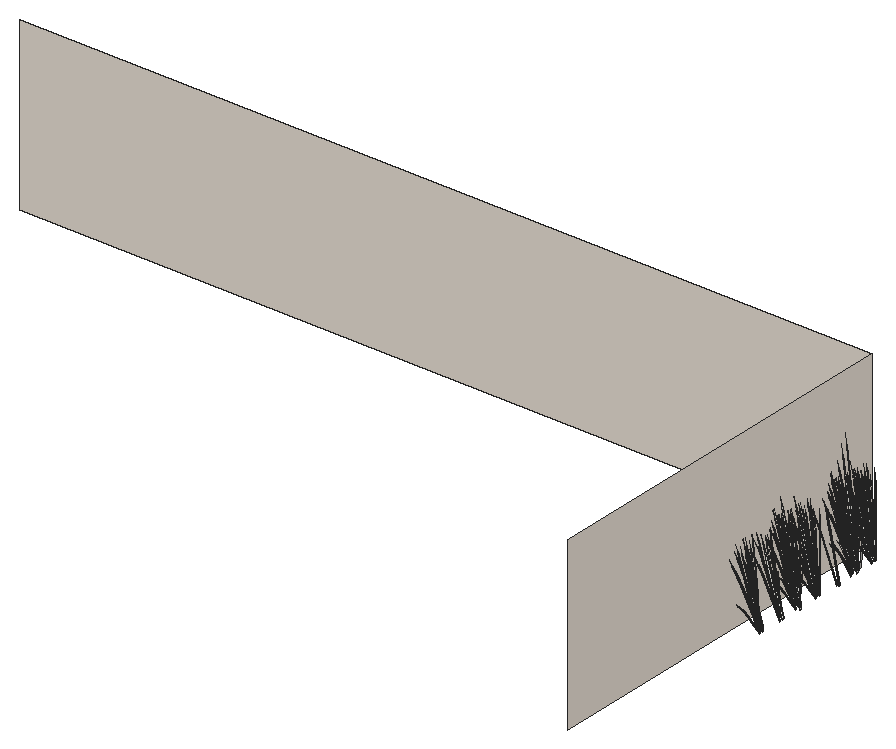
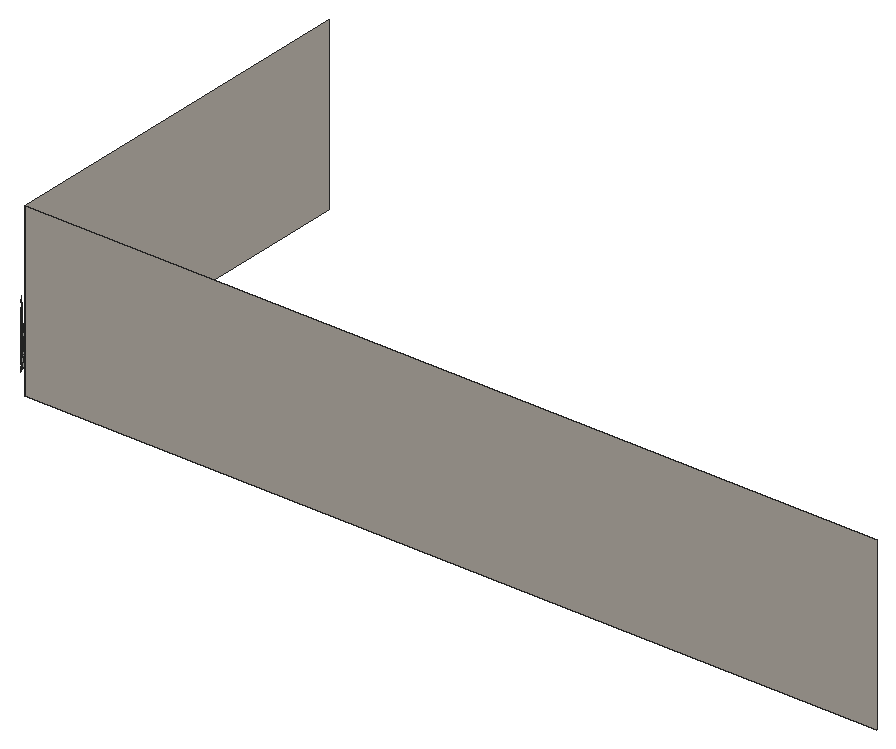
# SketchUp Ruby script. Lengths in inches.
U = 1.inch
M = Sketchup.active_model
def pt(a) = Geom::Point3d.new(a.map { |v| v * U })
def face(e, loops, mat)
  f = e.add_face(loops[0].map { |a| pt(a) })
  loops[1..].each { |l| e.add_face(l.map { |a| pt(a) }).erase! }
  f.material = f.back_material = mat if mat
  f
end
# faces: each face lists its corners as indices into pts; further lists are holes
def faces(e, pts, list, mat = nil) = list.each { |f| face(e, (f[0].is_a?(Array) ? f : [f]).map { |l| l.map { |i| pts[i] } }, mat) }
# xy, xz, yz: faces in a plane at the given z, y or x. An outline is a flat list of corners, or four numbers for a rectangle; further outlines are holes
def ring(l) = l.size == 4 ? [[l[0], l[1]], [l[2], l[1]], [l[2], l[3]], [l[0], l[3]]] : l.each_slice(2).to_a
def flat(e, list, mat, &to3) = list.each { |f| face(e, (f[0].is_a?(Array) ? f : [f]).map { |l| ring(l).map { |u, v| to3.(u, v) } }, mat) }
def xy(e, z, list, mat = nil) = flat(e, list, mat) { |x, y| [x, y, z] }
def xz(e, y, list, mat = nil) = flat(e, list, mat) { |x, z| [x, y, z] }
def yz(e, x, list, mat = nil) = flat(e, list, mat) { |y, z| [x, y, z] }
def lines(e, pts, list) = list.each { |a, b| e.add_line(pt(pts[a]), pt(pts[b])) }
# prism: a flat outline (further loops are holes) pulled along v
def prism(e, loops, v, mat = nil)
  f = face(e, loops, mat); d = Geom::Vector3d.new(v.map { |x| x * U })
  f.pushpull(f.normal.samedirection?(d) ? d.length : -d.length)
end
def box(e, o, s, mat = nil) = prism(e, [[o, [o[0] + s[0], o[1], o[2]], [o[0] + s[0], o[1] + s[1], o[2]], [o[0], o[1] + s[1], o[2]]]], [0, 0, s[2]], mat)
def at(x, y, z, deg = 0) = Geom::Transformation.translation(pt([x, y, z])) * Geom::Transformation.rotation(ORIGIN, Z_AXIS, deg.degrees)
def axes(o, x, y, z) = Geom::Transformation.new([*x, 0, *y, 0, *z, 0, *pt(o).to_a, 1])
def part(name) = M.definitions.add(name)
# library, detail: a bought-in or finely detailed component or shape, given as its bounding box
def library(name, o, s) = part(name).tap { |d| box(d.entities, o, s) }
def detail(e, o, s) = box(e.add_group.entities, o, s)
def put(e, d, t, mat = nil) = e.add_instance(d, t).tap { |i| i.material = mat if mat }
def group(e, t, mat = nil) = e.add_group.tap { |g| g.transformation = t; g.material = mat if mat }.entities
root = M.entities
M.materials.add("LightPink_Translucent").color = [144, 107, 117]
M.materials["LightPink_Translucent"].alpha = 0.75
M.materials.add("Marble_01_1K").color = [230, 221, 211]
c1 = part("blade")
p = [[2.15,0.21,22],[0,0.17,0],[0.09,0.45,0],[2.18,0.31,22],[2.29,0.31,22],[0.38,0.45,0],
  [2.48,0.24,33],[2.49,0.24,33],[2.48,0.22,33]]
faces(c1.entities,p,[[0,1,2,3],[4,5,2,3],[6,3,4,7],[8,0,3,6]])
c2 = part("seeds")
p = [[0.3,-0.1,1.38],[-0.01,-0.03,1.59],[-0.01,-0.03,0.03],[0.14,-0.07,-0.07],[0.29,-0.03,3],[0.15,0.01,3.11]]
faces(c2.entities,p,[[0,1,2,3],[1,0,4,5]],"LightPink_Translucent")
c3 = part("blade with seeds")
put(c3.entities,c1,at(0,0,0))
put(c3.entities,c2,axes([2.4,0.25,30.99],[1.5799,-0.05474,1.17369],[-0.12525,1.92788,0.29478],[-0.07173,-0.02425,1.56792]))
xz(root,432,[[0,-12,390,66]],"Marble_01_1K")
yz(root,390,[[258,-12,432,66]],"Marble_01_1K")
put(root,c3,axes([400.06,408.33,-8.39],[0.21212,-0.01231,1.59586],[-0.14072,0.53355,0.12904],[-0.3023,-0.033,0.68222]))
put(root,c3,axes([400.15,409.27,-8.39],[0.17745,-0.11497,1.59586],[0.14939,0.53127,0.12904],[-0.27857,0.12007,0.68222]))
put(root,c3,axes([399.6,410.18,-9.59],[0.17773,0.04462,1.33163],[0.11455,0.45576,-0.28638],[-0.24142,0.08531,0.56934]))
put(root,c3,axes([400.86,374.66,-8.39],[0.21212,-0.01231,1.59586],[-0.14072,0.53355,0.12904],[-0.3023,-0.033,0.68222]))
put(root,c3,axes([401.17,408.72,-8.89],[0.14537,-0.07863,1.64882],[0.05013,0.549,0.12904],[-0.31487,0.07285,0.5893]))
put(root,c3,axes([401.01,417.9375,-8.39],[0.21212,-0.01231,1.59586],[-0.14072,0.53355,0.12904],[-0.3023,-0.033,0.68222]))
put(root,c3,axes([401.14,385.52,-8.39],[0.21212,-0.01231,1.59586],[-0.14072,0.53355,0.12904],[-0.3023,-0.033,0.68222]))
put(root,c3,axes([399.61,409.09,-7.61],[-0.08351,0.07057,1.62908],[0.0071,0.51561,-0.25764],[-0.19143,0.06705,0.13065]))
put(root,c3,axes([400.69,407.84,-7.36],[-0.51122,-0.01309,-0.66157],[0.03434,-0.5511,0.07984],[-0.21658,-0.05816,0.93586]))
put(root,c3,axes([400.28,407.97,-9.59],[0.09985,0.15133,1.33163],[-0.23008,0.41134,-0.28638],[-0.23625,-0.09832,0.56934]))
put(root,c3,axes([399.875,408.79,-7.78],[-0.42502,-0.15163,-0.32977],[0.12396,-0.44238,0.42575],[-0.17112,0.04056,0.81462]))
put(root,c3,axes([400.95,375.6,-8.39],[0.17745,-0.11497,1.59586],[0.14939,0.53127,0.12904],[-0.27857,0.12007,0.68222]))
put(root,c3,axes([400.46,407.48,-8.39],[0.18996,0.09365,1.59586],[-0.39312,0.39287,0.12904],[-0.24502,-0.17723,0.68222]))
put(root,c3,axes([400.4,376.51,-9.59],[0.17773,0.04462,1.33163],[0.11455,0.45576,-0.28638],[-0.24142,0.08531,0.56934]))
put(root,c3,axes([401.1,418.875,-8.39],[0.17745,-0.11497,1.59586],[0.14939,0.53127,0.12904],[-0.27857,0.12007,0.68222]))
put(root,c3,axes([398.68,409.61,-7.62],[0.06527,0.01458,1.65179],[0.20191,0.48025,-0.15608],[-0.1336,0.12605,0.29231]))
put(root,c3,axes([400.16,409.02,-7.64],[-0.13855,0.49442,-0.47583],[-0.47502,-0.16947,-0.36857],[-0.19125,0.04534,0.91046]))
put(root,c3,axes([400.55,419.78,-9.59],[0.17773,0.04462,1.33163],[0.11455,0.45576,-0.28638],[-0.24142,0.08531,0.56934]))
put(root,c3,axes([401.23,386.46,-8.39],[0.17745,-0.11497,1.59586],[0.14939,0.53127,0.12904],[-0.27857,0.12007,0.68222]))
put(root,c3,axes([401.97,375.05,-8.89],[0.14537,-0.07863,1.64882],[0.05013,0.549,0.12904],[-0.31487,0.07285,0.5893]))
put(root,c3,axes([400.52,407.95,-7.64],[-0.37135,0.36005,-0.47583],[-0.32522,-0.38035,-0.36857],[-0.18868,-0.05478,0.91046]))
put(root,c3,axes([399.93,408.99,-10.61],[0.01297,0.08566,1.6421],[-0.26146,0.44735,-0.25086],[-0.18572,-0.02255,0.2797]))
put(root,c3,axes([400.68,387.37,-9.59],[0.17773,0.04462,1.33163],[0.11455,0.45576,-0.28638],[-0.24142,0.08531,0.56934]))
put(root,c3,axes([402.12,418.32,-8.89],[0.14537,-0.07863,1.64882],[0.05013,0.549,0.12904],[-0.31487,0.07285,0.5893]))
put(root,c3,axes([400,406.94,-7.62],[0.03791,0.05424,1.65179],[-0.18278,0.48761,-0.15608],[-0.18511,0.00353,0.29231]))
put(root,c3,axes([401.91,352.82,-8.39],[0.21212,-0.01231,1.59586],[-0.14072,0.53355,0.12904],[-0.3023,-0.033,0.68222]))
put(root,c3,axes([399.23,411.13,-9.42],[0.21313,-0.24635,1.06958],[0.0841,0.38999,0.78586],[-0.15402,0.06983,0.23558]))
put(root,c3,axes([402.25,385.91,-8.89],[0.14537,-0.07863,1.64882],[0.05013,0.549,0.12904],[-0.31487,0.07285,0.5893]))
put(root,c3,axes([400.42,406.62,-7.61],[-0.11004,-0.00384,1.62908],[-0.35032,0.38367,-0.25764],[-0.18692,-0.07839,0.13065]))
put(root,c3,axes([400.41,375.41,-7.61],[-0.08351,0.07057,1.62908],[0.0071,0.51561,-0.25764],[-0.19143,0.06705,0.13065]))
put(root,c3,axes([401.5,374.17,-7.36],[-0.51122,-0.01309,-0.66157],[0.03434,-0.5511,0.07984],[-0.21658,-0.05816,0.93586]))
put(root,c3,axes([399.97,408.74,-7.59],[0.14449,-0.4956,0.447],[0.47502,0.16947,0.36857],[-0.1868,0.02978,0.92496]))
put(root,c3,axes([401.09,374.3,-9.59],[0.09985,0.15133,1.33163],[-0.23008,0.41134,-0.28638],[-0.23625,-0.09832,0.56934]))
put(root,c3,axes([400.14,408.6,-7.3125],[0.25732,0.49218,-0.11324],[-0.45669,0.24187,-0.62851],[-0.19245,0.06494,0.95501]))
put(root,c3,axes([400.72,407.57,-7.3125],[-0.02738,0.55277,-0.11324],[-0.51847,-0.01511,-0.62851],[-0.19968,-0.0384,0.95501]))
put(root,c3,axes([400.56,418.6875,-7.61],[-0.08351,0.07057,1.62908],[0.0071,0.51561,-0.25764],[-0.19143,0.06705,0.13065]))
put(root,c3,axes([400.39,407.61,-7.78],[-0.29098,-0.34031,-0.32977],[0.33226,-0.32215,0.42575],[-0.16881,-0.04902,0.81462]))
put(root,c3,axes([400.68,375.12,-7.78],[-0.42502,-0.15163,-0.32977],[0.12396,-0.44238,0.42575],[-0.17112,0.04056,0.81462]))
put(root,c3,axes([401.65,417.44,-7.36],[-0.51122,-0.01309,-0.66157],[0.03434,-0.5511,0.07984],[-0.21658,-0.05816,0.93586]))
put(root,c3,axes([399.9375,408.61,-7.6],[-0.18783,-0.37061,0.05988],[0.34252,-0.1814,0.47138],[-0.15099,0.03579,0.71878]))
put(root,c3,axes([401.27,373.81,-8.39],[0.18996,0.09365,1.59586],[-0.39312,0.39287,0.12904],[-0.24502,-0.17723,0.68222]))
put(root,c3,axes([400.8,409.63,-8.39],[0.12773,-0.16701,1.59586],[0.32252,0.4508,0.12904],[-0.22121,0.20529,0.68222]))
put(root,c3,axes([401.23,417.57,-9.59],[0.09985,0.15133,1.33163],[-0.23008,0.41134,-0.28638],[-0.23625,-0.09832,0.56934]))
put(root,c3,axes([400.03,410.07,-7.78],[-0.44516,0.07768,-0.32977],[-0.11755,-0.44407,0.42575],[-0.12757,0.11927,0.81462]))
put(root,c3,axes([400.69,386.27,-7.61],[-0.08351,0.07057,1.62908],[0.0071,0.51561,-0.25764],[-0.19143,0.06705,0.13065]))
put(root,c3,axes([401.78,385.03,-7.36],[-0.51122,-0.01309,-0.66157],[0.03434,-0.5511,0.07984],[-0.21658,-0.05816,0.93586]))
put(root,c3,axes([400.82,418.39,-7.78],[-0.42502,-0.15163,-0.32977],[0.12396,-0.44238,0.42575],[-0.17112,0.04056,0.81462]))
put(root,c3,axes([399.79,411.39,-10.61],[0.0686,0.0543,1.6421],[0.11632,0.50315,-0.25086],[-0.15204,0.10729,0.2797]))
put(root,c3,axes([401.41,417.08,-8.39],[0.18996,0.09365,1.59586],[-0.39312,0.39287,0.12904],[-0.24502,-0.17723,0.68222]))
put(root,c3,axes([401.37,385.16,-9.59],[0.09985,0.15133,1.33163],[-0.23008,0.41134,-0.28638],[-0.23625,-0.09832,0.56934]))
put(root,c3,axes([399.6875,408.43,-9.42],[0.3265,-0.03889,1.06958],[-0.20711,0.3427,0.78586],[-0.16135,-0.05141,0.23558]))
put(root,c3,axes([399.48,375.9375,-7.62],[0.06527,0.01458,1.65179],[0.20191,0.48025,-0.15608],[-0.1336,0.12605,0.29231]))
put(root,c3,axes([400.97,375.35,-7.64],[-0.13855,0.49442,-0.47583],[-0.47502,-0.16947,-0.36857],[-0.19125,0.04534,0.91046]))
put(root,c3,axes([402.43,364.02,-8.39],[0.21212,-0.01231,1.59586],[-0.14072,0.53355,0.12904],[-0.3023,-0.033,0.68222]))
put(root,c3,axes([402,353.75,-8.39],[0.17745,-0.11497,1.59586],[0.14939,0.53127,0.12904],[-0.27857,0.12007,0.68222]))
put(root,c3,axes([400.96,385.98,-7.78],[-0.42502,-0.15163,-0.32977],[0.12396,-0.44238,0.42575],[-0.17112,0.04056,0.81462]))
put(root,c3,axes([401.55,384.66,-8.39],[0.18996,0.09365,1.59586],[-0.39312,0.39287,0.12904],[-0.24502,-0.17723,0.68222]))
put(root,c3,axes([401.33,374.28,-7.64],[-0.37135,0.36005,-0.47583],[-0.32522,-0.38035,-0.36857],[-0.18868,-0.05478,0.91046]))
put(root,c3,axes([400.73,375.32,-10.61],[0.01297,0.08566,1.6421],[-0.26146,0.44735,-0.25086],[-0.18572,-0.02255,0.2797]))
put(root,c3,axes([399.63,419.21,-7.62],[0.06527,0.01458,1.65179],[0.20191,0.48025,-0.15608],[-0.1336,0.12605,0.29231]))
put(root,c3,axes([400.09,409.97,-7.59],[-0.12683,-0.50025,0.447],[0.49754,-0.08682,0.36857],[-0.14663,0.11765,0.92496]))
put(root,c3,axes([401.12,418.62,-7.64],[-0.13855,0.49442,-0.47583],[-0.47502,-0.16947,-0.36857],[-0.19125,0.04534,0.91046]))
put(root,c3,axes([401.45,354.66,-9.59],[0.17773,0.04462,1.33163],[0.11455,0.45576,-0.28638],[-0.24142,0.08531,0.56934]))
put(root,c3,axes([400.34,407.48,-7.26],[0.42234,-0.40113,0.50064],[0.36424,0.42599,0.4128],[-0.19815,-0.07399,1.03595]))
put(root,c3,axes([401.48,417.55,-7.64],[-0.37135,0.36005,-0.47583],[-0.32522,-0.38035,-0.36857],[-0.18868,-0.05478,0.91046]))
put(root,c3,axes([400.81,373.27,-7.62],[0.03791,0.05424,1.65179],[-0.18278,0.48761,-0.15608],[-0.18511,0.00353,0.29231]))
put(root,c3,axes([400.875,418.59,-10.61],[0.01297,0.08566,1.6421],[-0.26146,0.44735,-0.25086],[-0.18572,-0.02255,0.2797]))
put(root,c3,axes([399.76,386.79,-7.62],[0.06527,0.01458,1.65179],[0.20191,0.48025,-0.15608],[-0.1336,0.12605,0.29231]))
put(root,c3,axes([399.99,409.875,-7.6],[-0.35109,-0.22859,0.05988],[0.2044,-0.32553,0.47138],[-0.11256,0.10524,0.71878]))
put(root,c3,axes([401.25,386.2,-7.64],[-0.13855,0.49442,-0.47583],[-0.47502,-0.16947,-0.36857],[-0.19125,0.04534,0.91046]))
put(root,c3,axes([403.02,353.2,-8.89],[0.14537,-0.07863,1.64882],[0.05013,0.549,0.12904],[-0.31487,0.07285,0.5893]))
put(root,c3,axes([400.03,377.46,-9.42],[0.21313,-0.24635,1.06958],[0.0841,0.38999,0.78586],[-0.15402,0.06983,0.23558]))
put(root,c3,axes([401.61,385.14,-7.64],[-0.37135,0.36005,-0.47583],[-0.32522,-0.38035,-0.36857],[-0.18868,-0.05478,0.91046]))
put(root,c3,axes([401.23,372.94,-7.61],[-0.11004,-0.00384,1.62908],[-0.35032,0.38367,-0.25764],[-0.18692,-0.07839,0.13065]))
put(root,c3,axes([401.01,386.17,-10.61],[0.01297,0.08566,1.6421],[-0.26146,0.44735,-0.25086],[-0.18572,-0.02255,0.2797]))
put(root,c3,axes([400.95,416.54,-7.62],[0.03791,0.05424,1.65179],[-0.18278,0.48761,-0.15608],[-0.18511,0.00353,0.29231]))
put(root,c3,axes([400.7,410.04,-8.39],[0.09522,-0.18683,1.59586],[0.39947,0.38663,0.12904],[-0.18021,0.24097,0.68222]))
put(root,c3,axes([400.78,375.07,-7.59],[0.14449,-0.4956,0.447],[0.47502,0.16947,0.36857],[-0.1868,0.02978,0.92496]))
put(root,c3,axes([400.18,420.73,-9.42],[0.21313,-0.24635,1.06958],[0.0841,0.38999,0.78586],[-0.15402,0.06983,0.23558]))
put(root,c3,axes([400.95,374.92,-7.3125],[0.25732,0.49218,-0.11324],[-0.45669,0.24187,-0.62851],[-0.19245,0.06494,0.95501]))
put(root,c3,axes([401.09,384.13,-7.62],[0.03791,0.05424,1.65179],[-0.18278,0.48761,-0.15608],[-0.18511,0.00353,0.29231]))
put(root,c3,axes([401.375,416.22,-7.61],[-0.11004,-0.00384,1.62908],[-0.35032,0.38367,-0.25764],[-0.18692,-0.07839,0.13065]))
put(root,c3,axes([402.52,364.96,-8.39],[0.17745,-0.11497,1.59586],[0.14939,0.53127,0.12904],[-0.27857,0.12007,0.68222]))
put(root,c3,axes([401.52,373.9,-7.3125],[-0.02738,0.55277,-0.11324],[-0.51847,-0.01511,-0.62851],[-0.19968,-0.0384,0.95501]))
put(root,c3,axes([401.19,373.9375,-7.78],[-0.29098,-0.34031,-0.32977],[0.33226,-0.32215,0.42575],[-0.16881,-0.04902,0.81462]))
put(root,c3,axes([400.74,374.93,-7.6],[-0.18783,-0.37061,0.05988],[0.34252,-0.1814,0.47138],[-0.15099,0.03579,0.71878]))
put(root,c3,axes([400.32,408.74,-7.3],[0.42502,0.15163,0.32977],[-0.12396,0.44238,-0.42575],[-0.17112,0.04056,0.81462]))
put(root,c3,axes([400.31,388.32,-9.42],[0.21313,-0.24635,1.06958],[0.0841,0.38999,0.78586],[-0.15402,0.06983,0.23558]))
put(root,c3,axes([400.92,418.34,-7.59],[0.14449,-0.4956,0.447],[0.47502,0.16947,0.36857],[-0.1868,0.02978,0.92496]))
put(root,c3,axes([401.6,375.96,-8.39],[0.12773,-0.16701,1.59586],[0.32252,0.4508,0.12904],[-0.22121,0.20529,0.68222]))
put(root,c3,axes([400.83,376.4,-7.78],[-0.44516,0.07768,-0.32977],[-0.11755,-0.44407,0.42575],[-0.12757,0.11927,0.81462]))
put(root,c3,axes([401.97,365.86,-9.59],[0.17773,0.04462,1.33163],[0.11455,0.45576,-0.28638],[-0.24142,0.08531,0.56934]))
put(root,c3,axes([401.46,353.57,-7.61],[-0.08351,0.07057,1.62908],[0.0071,0.51561,-0.25764],[-0.19143,0.06705,0.13065]))
put(root,c3,axes([401.09,418.2,-7.3125],[0.25732,0.49218,-0.11324],[-0.45669,0.24187,-0.62851],[-0.19245,0.06494,0.95501]))
put(root,c3,axes([401.51,383.8,-7.61],[-0.11004,-0.00384,1.62908],[-0.35032,0.38367,-0.25764],[-0.18692,-0.07839,0.13065]))
put(root,c3,axes([402.55,352.32,-7.36],[-0.51122,-0.01309,-0.66157],[0.03434,-0.5511,0.07984],[-0.21658,-0.05816,0.93586]))
put(root,c3,axes([400.4,410.12,-7.64],[0.13138,0.49631,-0.47583],[-0.49754,0.08682,-0.36857],[-0.14258,0.13331,0.91046]))
put(root,c3,axes([401.67,417.17,-7.3125],[-0.02738,0.55277,-0.11324],[-0.51847,-0.01511,-0.62851],[-0.19968,-0.0384,0.95501]))
put(root,c3,axes([401.34,417.21,-7.78],[-0.29098,-0.34031,-0.32977],[0.33226,-0.32215,0.42575],[-0.16881,-0.04902,0.81462]))
put(root,c3,axes([400.89,418.21,-7.6],[-0.18783,-0.37061,0.05988],[0.34252,-0.1814,0.47138],[-0.15099,0.03579,0.71878]))
put(root,c3,axes([402.14,352.45,-9.59],[0.09985,0.15133,1.33163],[-0.23008,0.41134,-0.28638],[-0.23625,-0.09832,0.56934]))
put(root,c3,axes([400.54,407.48,-7.6],[0.02575,-0.41332,0.05988],[0.38885,0.01133,0.47138],[-0.14895,-0.04325,0.71878]))
put(root,c3,axes([400.59,377.71,-10.61],[0.0686,0.0543,1.6421],[0.11632,0.50315,-0.25086],[-0.15204,0.10729,0.2797]))
put(root,c3,axes([399.62,411.01,-7.61],[-0.01271,0.10756,1.62908],[0.36076,0.37419,-0.25764],[-0.09444,0.17695,0.13065]))
put(root,c3,axes([401.06,385.92,-7.59],[0.14449,-0.4956,0.447],[0.47502,0.16947,0.36857],[-0.1868,0.02978,0.92496]))
put(root,c3,axes([401.75,419.23,-8.39],[0.12773,-0.16701,1.59586],[0.32252,0.4508,0.12904],[-0.22121,0.20529,0.68222]))
put(root,c3,axes([400.49,374.75,-9.42],[0.3265,-0.03889,1.06958],[-0.20711,0.3427,0.78586],[-0.16135,-0.05141,0.23558]))
put(root,c3,axes([400.98,419.67,-7.78],[-0.44516,0.07768,-0.32977],[-0.11755,-0.44407,0.42575],[-0.12757,0.11927,0.81462]))
put(root,c3,axes([401.64,409.76,-10.08],[-0.53199,-0.08911,-0.58063],[0.11226,-0.54969,-0.15239],[-0.15876,-0.06661,1.28164]))
put(root,c3,axes([401.23,385.78,-7.3125],[0.25732,0.49218,-0.11324],[-0.45669,0.24187,-0.62851],[-0.19245,0.06494,0.95501]))
put(root,c3,axes([401.73,406.77,-6.94],[-0.34131,0.52108,-0.12682],[-0.49429,-0.3002,-0.70393],[-0.17182,-0.14722,1.06961]))
put(root,c3,axes([401.73,353.27,-7.78],[-0.42502,-0.15163,-0.32977],[0.12396,-0.44238,0.42575],[-0.17112,0.04056,0.81462]))
put(root,c3,axes([401.8,384.76,-7.3125],[-0.02738,0.55277,-0.11324],[-0.51847,-0.01511,-0.62851],[-0.19968,-0.0384,0.95501]))
put(root,c3,axes([403.54,364.4,-8.89],[0.14537,-0.07863,1.64882],[0.05013,0.549,0.12904],[-0.31487,0.07285,0.5893]))
put(root,c3,axes([401.47,384.8,-7.78],[-0.29098,-0.34031,-0.32977],[0.33226,-0.32215,0.42575],[-0.16881,-0.04902,0.81462]))
put(root,c3,axes([402.32,351.96,-8.39],[0.18996,0.09365,1.59586],[-0.39312,0.39287,0.12904],[-0.24502,-0.17723,0.68222]))
put(root,c3,axes([401.02,385.79,-7.6],[-0.18783,-0.37061,0.05988],[0.34252,-0.1814,0.47138],[-0.15099,0.03579,0.71878]))
put(root,c3,axes([400.8,407.79,-7.3],[0.29098,0.34031,0.32977],[-0.33226,0.32215,-0.42575],[-0.16881,-0.04902,0.81462]))
put(root,c3,axes([400.74,420.99,-10.61],[0.0686,0.0543,1.6421],[0.11632,0.50315,-0.25086],[-0.15204,0.10729,0.2797]))
put(root,c3,axes([401.88,386.82,-8.39],[0.12773,-0.16701,1.59586],[0.32252,0.4508,0.12904],[-0.22121,0.20529,0.68222]))
put(root,c3,axes([401.11,387.25,-7.78],[-0.44516,0.07768,-0.32977],[-0.11755,-0.44407,0.42575],[-0.12757,0.11927,0.81462]))
put(root,c3,axes([400.64,418.03,-9.42],[0.3265,-0.03889,1.06958],[-0.20711,0.3427,0.78586],[-0.16135,-0.05141,0.23558]))
put(root,c3,axes([400.89,376.3,-7.59],[-0.12683,-0.50025,0.447],[0.49754,-0.08682,0.36857],[-0.14663,0.11765,0.92496]))
put(root,c3,axes([401.58,407.1875,-7.36],[-0.43608,-0.26272,-0.66157],[0.30991,-0.46038,0.07984],[-0.158,-0.15687,0.93586]))
put(root,c3,axes([401.38,407.2,-7.64],[-0.50465,0.12921,-0.47583],[-0.08828,-0.48932,-0.36857],[-0.13555,-0.14022,0.91046]))
put(root,c3,axes([400.87,388.57,-10.61],[0.0686,0.0543,1.6421],[0.11632,0.50315,-0.25086],[-0.15204,0.10729,0.2797]))
put(root,c3,axes([401.15,373.8125,-7.26],[0.42234,-0.40113,0.50064],[0.36424,0.42599,0.4128],[-0.19815,-0.07399,1.03595]))
put(root,c3,axes([400.53,354.09,-7.62],[0.06527,0.01458,1.65179],[0.20191,0.48025,-0.15608],[-0.1336,0.12605,0.29231]))
put(root,c3,axes([403.45,395.21,-8.39],[0.21212,-0.01231,1.59586],[-0.14072,0.53355,0.12904],[-0.3023,-0.033,0.68222]))
put(root,c3,axes([402.02,353.5,-7.64],[-0.13855,0.49442,-0.47583],[-0.47502,-0.16947,-0.36857],[-0.19125,0.04534,0.91046]))
put(root,c3,axes([400.77,385.61,-9.42],[0.3265,-0.03889,1.06958],[-0.20711,0.3427,0.78586],[-0.16135,-0.05141,0.23558]))
put(root,c3,axes([400.79,376.2,-7.6],[-0.35109,-0.22859,0.05988],[0.2044,-0.32553,0.47138],[-0.11256,0.10524,0.71878]))
put(root,c3,axes([401.04,419.57,-7.59],[-0.12683,-0.50025,0.447],[0.49754,-0.08682,0.36857],[-0.14663,0.11765,0.92496]))
put(root,c3,axes([400.9375,410.8,-10.12],[-0.47863,-0.27177,-0.46235],[0.28609,-0.48733,0],[-0.10901,-0.0619,1.46668]))
put(root,c3,axes([402.38,352.43,-7.64],[-0.37135,0.36005,-0.47583],[-0.32522,-0.38035,-0.36857],[-0.18868,-0.05478,0.91046]))
put(root,c3,axes([400.73,406.76,-10.61],[-0.04954,0.0716,1.6421],[-0.50062,0.15438,-0.25086],[-0.12094,-0.14044,0.2797]))
put(root,c3,axes([400.16,409.77,-7.3125],[0.47307,0.29971,-0.11324],[-0.27254,0.43404,-0.62851],[-0.13365,0.15087,0.95501]))
put(root,c3,axes([401.78,353.47,-10.61],[0.01297,0.08566,1.6421],[-0.26146,0.44735,-0.25086],[-0.18572,-0.02255,0.2797]))
put(root,c3,axes([401.98,364.77,-7.61],[-0.08351,0.07057,1.62908],[0.0071,0.51561,-0.25764],[-0.19143,0.06705,0.13065]))
put(root,c3,axes([401.29,417.08,-7.26],[0.42234,-0.40113,0.50064],[0.36424,0.42599,0.4128],[-0.19815,-0.07399,1.03595]))
put(root,c3,axes([403.06,363.52,-7.36],[-0.51122,-0.01309,-0.66157],[0.03434,-0.5511,0.07984],[-0.21658,-0.05816,0.93586]))
put(root,c3,axes([401.17,387.16,-7.59],[-0.12683,-0.50025,0.447],[0.49754,-0.08682,0.36857],[-0.14663,0.11765,0.92496]))
put(root,c3,axes([400.9375,419.48,-7.6],[-0.35109,-0.22859,0.05988],[0.2044,-0.32553,0.47138],[-0.11256,0.10524,0.71878]))
put(root,c3,axes([401.23,411.13,-9.79],[-0.31974,0.54466,0],[-0.53494,-0.30375,-0.48057],[-0.12184,-0.06918,1.52448]))
put(root,c3,axes([401.51,376.37,-8.39],[0.09522,-0.18683,1.59586],[0.39947,0.38663,0.12904],[-0.18021,0.24097,0.68222]))
put(root,c3,axes([402.65,363.66,-9.59],[0.09985,0.15133,1.33163],[-0.23008,0.41134,-0.28638],[-0.23625,-0.09832,0.56934]))
put(root,c3,axes([401.86,351.42,-7.62],[0.03791,0.05424,1.65179],[-0.18278,0.48761,-0.15608],[-0.18511,0.00353,0.29231]))
put(root,c3,axes([401.43,384.67,-7.26],[0.42234,-0.40113,0.50064],[0.36424,0.42599,0.4128],[-0.19815,-0.07399,1.03595]))
put(root,c3,axes([402.24,364.48,-7.78],[-0.42502,-0.15163,-0.32977],[0.12396,-0.44238,0.42575],[-0.17112,0.04056,0.81462]))
put(root,c3,axes([401.07,387.0625,-7.6],[-0.35109,-0.22859,0.05988],[0.2044,-0.32553,0.47138],[-0.11256,0.10524,0.71878]))
put(root,c3,axes([402.83,363.16,-8.39],[0.18996,0.09365,1.59586],[-0.39312,0.39287,0.12904],[-0.24502,-0.17723,0.68222]))
put(root,c3,axes([401.65,419.64,-8.39],[0.09522,-0.18683,1.59586],[0.39947,0.38663,0.12904],[-0.18021,0.24097,0.68222]))
put(root,c3,axes([401.125,375.07,-7.3],[0.42502,0.15163,0.32977],[-0.12396,0.44238,-0.42575],[-0.17112,0.04056,0.81462]))
put(root,c3,axes([401.08,355.61,-9.42],[0.21313,-0.24635,1.06958],[0.0841,0.38999,0.78586],[-0.15402,0.06983,0.23558]))
put(root,c3,axes([402.28,351.1,-7.61],[-0.11004,-0.00384,1.62908],[-0.35032,0.38367,-0.25764],[-0.18692,-0.07839,0.13065]))
put(root,c3,axes([399.38,411.07,-6.74],[0.45129,0.14509,-0.06041],[-0.13882,0.44656,-0.27392],[-0.07381,0.0678,0.90349]))
put(root,c3,axes([401.2,376.45,-7.64],[0.13138,0.49631,-0.47583],[-0.49754,0.08682,-0.36857],[-0.14258,0.13331,0.91046]))
put(root,c3,axes([401.79,387.23,-8.39],[0.09522,-0.18683,1.59586],[0.39947,0.38663,0.12904],[-0.18021,0.24097,0.68222]))
put(root,c3,axes([400.39,409.81,-7.3],[0.44516,-0.07768,0.32977],[0.11755,0.44407,-0.42575],[-0.12757,0.11927,0.81462]))
put(root,c3,axes([401.83,353.22,-7.59],[0.14449,-0.4956,0.447],[0.47502,0.16947,0.36857],[-0.1868,0.02978,0.92496]))
put(root,c3,axes([401.34,373.81,-7.6],[0.02575,-0.41332,0.05988],[0.38885,0.01133,0.47138],[-0.14895,-0.04325,0.71878]))
put(root,c3,axes([401.27,418.35,-7.3],[0.42502,0.15163,0.32977],[-0.12396,0.44238,-0.42575],[-0.17112,0.04056,0.81462]))
put(root,c3,axes([401.05,365.29,-7.62],[0.06527,0.01458,1.65179],[0.20191,0.48025,-0.15608],[-0.1336,0.12605,0.29231]))
put(root,c3,axes([400.42,377.34,-7.61],[-0.01271,0.10756,1.62908],[0.36076,0.37419,-0.25764],[-0.09444,0.17695,0.13065]))
put(root,c3,axes([402.53,364.7,-7.64],[-0.13855,0.49442,-0.47583],[-0.47502,-0.16947,-0.36857],[-0.19125,0.04534,0.91046]))
put(root,c3,axes([403.54,396.15,-8.39],[0.17745,-0.11497,1.59586],[0.14939,0.53127,0.12904],[-0.27857,0.12007,0.68222]))
put(root,c3,axes([402,353.08,-7.3125],[0.25732,0.49218,-0.11324],[-0.45669,0.24187,-0.62851],[-0.19245,0.06494,0.95501]))
put(root,c3,axes([402.58,352.05,-7.3125],[-0.02738,0.55277,-0.11324],[-0.51847,-0.01511,-0.62851],[-0.19968,-0.0384,0.95501]))
put(root,c3,axes([400.65,411.92,-9.59],[0.16138,-0.08575,1.33163],[0.39845,0.25854,-0.28638],[-0.1186,0.22371,0.56934]))
put(root,c3,axes([402.44,376.09,-10.08],[-0.53199,-0.08911,-0.58063],[0.11226,-0.54969,-0.15239],[-0.15876,-0.06661,1.28164]))
put(root,c3,axes([402.54,373.09,-6.94],[-0.34131,0.52108,-0.12682],[-0.49429,-0.3002,-0.70393],[-0.17182,-0.14722,1.06961]))
put(root,c3,axes([402.24,352.09,-7.78],[-0.29098,-0.34031,-0.32977],[0.33226,-0.32215,0.42575],[-0.16881,-0.04902,0.81462]))
put(root,c3,axes([401.35,419.72,-7.64],[0.13138,0.49631,-0.47583],[-0.49754,0.08682,-0.36857],[-0.14258,0.13331,0.91046]))
put(root,c3,axes([401.79,353.09,-7.6],[-0.18783,-0.37061,0.05988],[0.34252,-0.1814,0.47138],[-0.15099,0.03579,0.71878]))
put(root,c3,axes([400.42,407.03,-10.02],[-0.14753,0.44383,-0.03625],[-0.45406,-0.13653,-0.16435],[-0.06894,-0.07259,0.54209]))
put(root,c3,axes([402.9,363.64,-7.64],[-0.37135,0.36005,-0.47583],[-0.32522,-0.38035,-0.36857],[-0.18868,-0.05478,0.91046]))
put(root,c3,axes([402.99,397.05,-9.59],[0.17773,0.04462,1.33163],[0.11455,0.45576,-0.28638],[-0.24142,0.08531,0.56934]))
